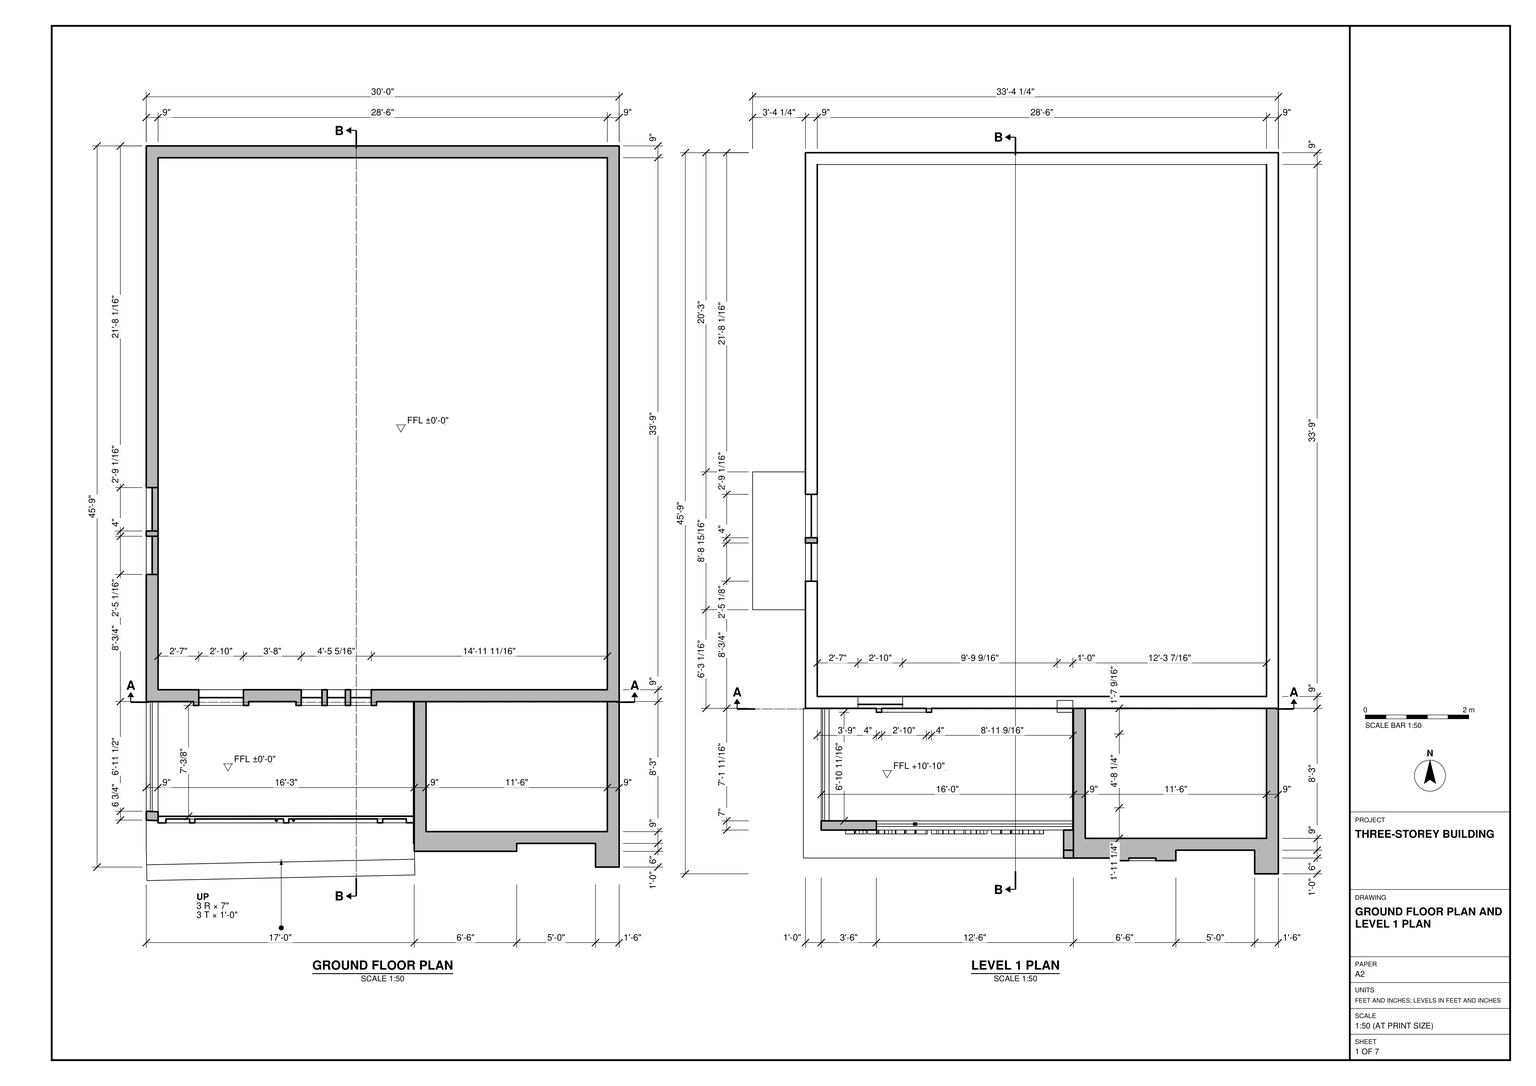
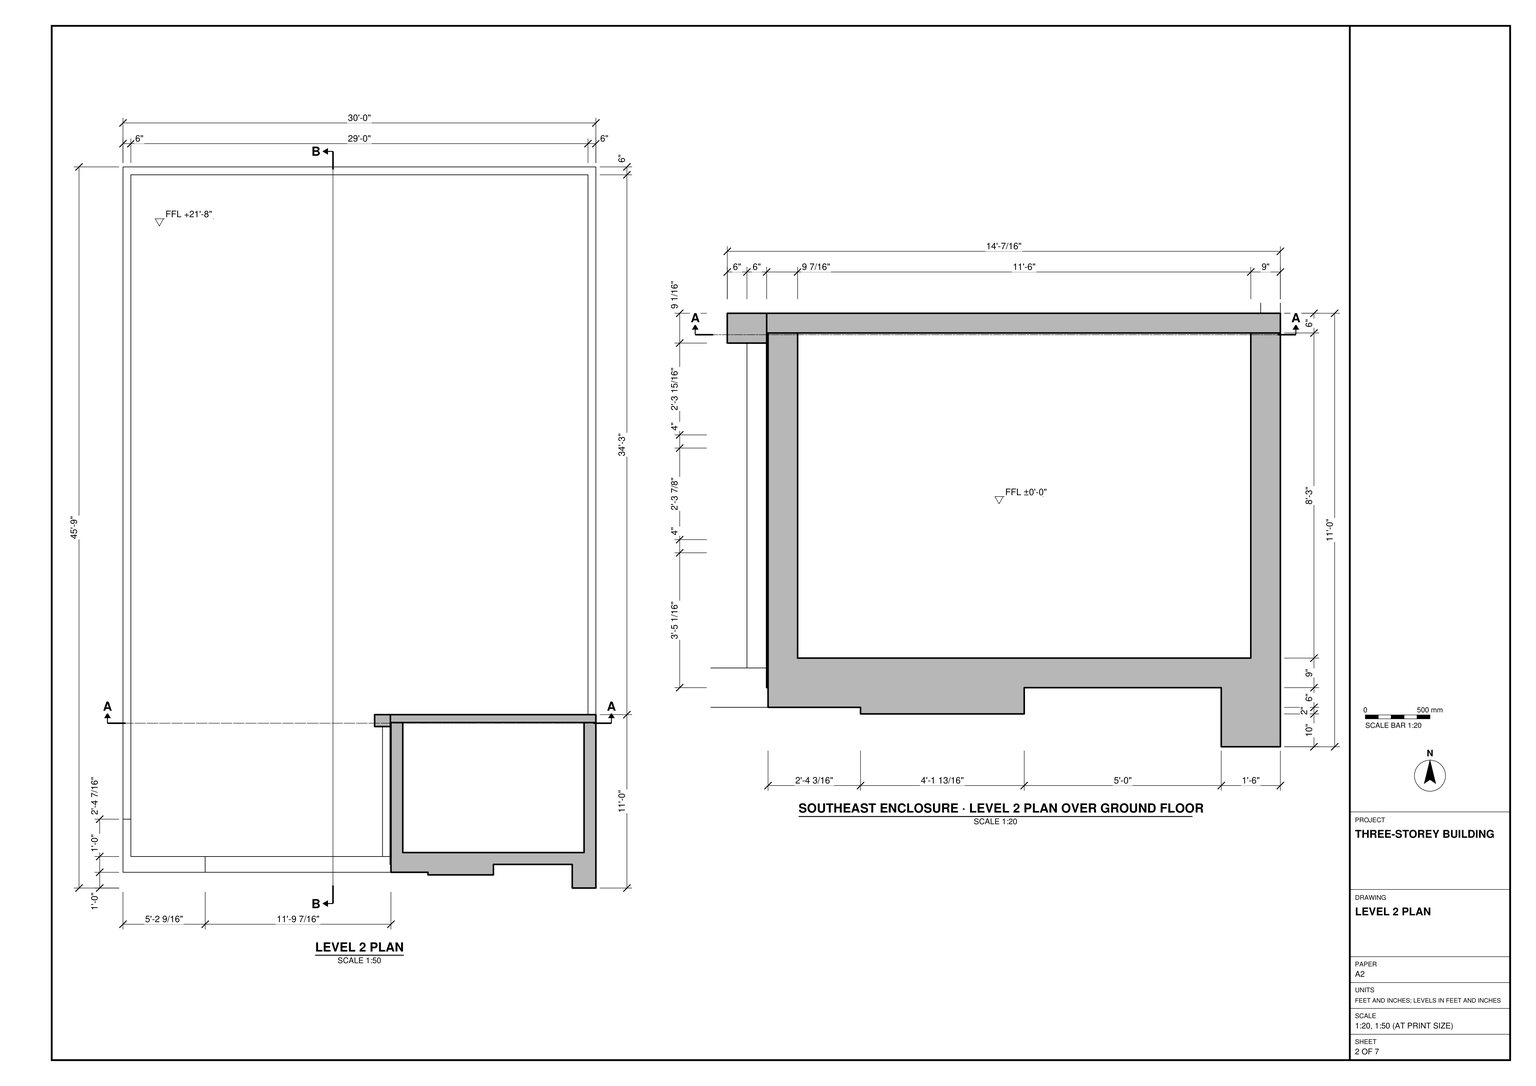
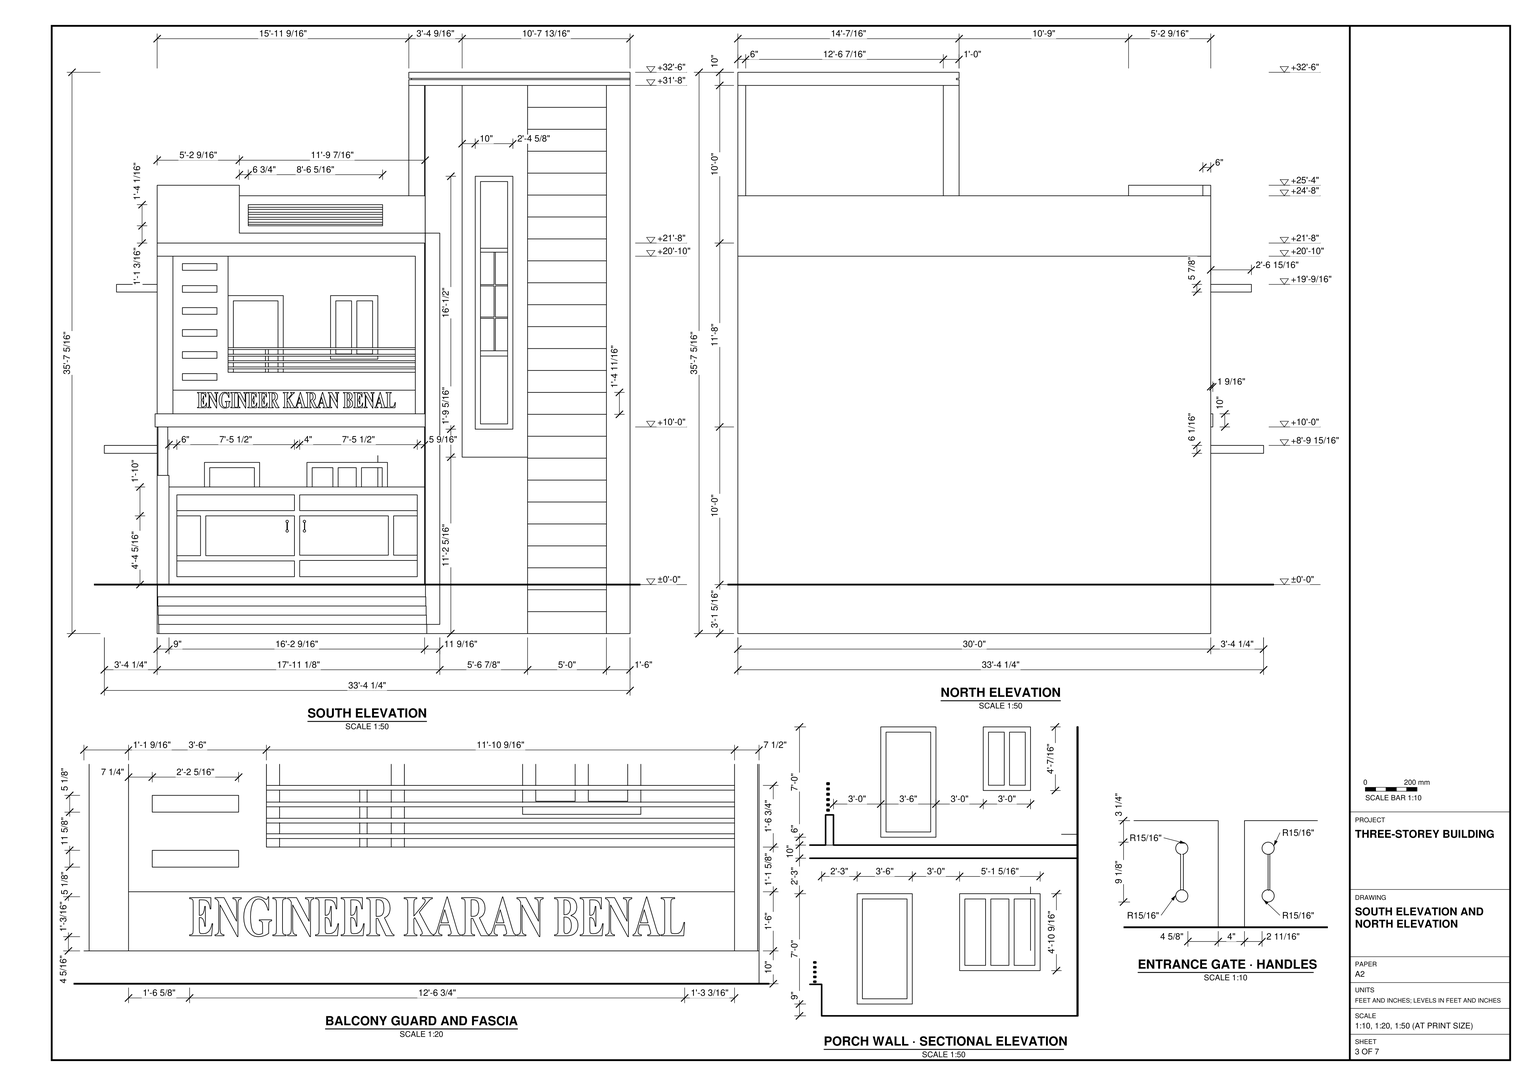
Build the three-storey building in SketchUp from task_files/diagram_01.pdf. Work in feet and inches. The complete model measures 33'-4 1/4" east to west, 49'-7 1/4" north to south and 35'-7 5/16" from the bottom of the base to the top of the roof. Set the ground floor at ±0'-0", Level 1 at +10'-0" and Level 2 at +21'-8".

Use the plans to lay out the rectangular main floor plates and the two bays on the south front. Keep the main floor areas open as drawn. Model the base, floor slabs, exterior walls, side projections and framed openings, using the wall thicknesses shown. In the western bay, build the entrance steps, double-leaf gate and covered porch. Place the balcony above the porch, with its solid fascia, horizontal guard rails and slotted end screen. Set the doors and windows in the walls behind the porch and balcony. In the eastern bay, carry the enclosure up past the terrace and reproduce the tall framed opening and adjacent horizontal joints on its south face. Finish the terrace with its parapets and the taller enclosure with its projecting flat roof cap.

Keep walls, slabs, roofs and each furniture or joinery piece shown in separate groups or components, and use components for repeated parts. Any decor or loose items shown may be suitable library components. Save one SketchUp model as output_files/three_storey_building_with_a_porch_and_roof_terrace.skp.

# SketchUp Ruby script. Lengths in inches.
U = 1.inch
M = Sketchup.active_model
def pt(a) = Geom::Point3d.new(a.map { |v| v * U })
def face(e, loops, mat)
  f = e.add_face(loops[0].map { |a| pt(a) })
  loops[1..].each { |l| e.add_face(l.map { |a| pt(a) }).erase! }
  f.material = f.back_material = mat if mat
  f
end
# faces: each face lists its corners as indices into pts; further lists are holes
def faces(e, pts, list, mat = nil) = list.each { |f| face(e, (f[0].is_a?(Array) ? f : [f]).map { |l| l.map { |i| pts[i] } }, mat) }
# xy, xz, yz: faces in a plane at the given z, y or x. An outline is a flat list of corners, or four numbers for a rectangle; further outlines are holes
def ring(l) = l.size == 4 ? [[l[0], l[1]], [l[2], l[1]], [l[2], l[3]], [l[0], l[3]]] : l.each_slice(2).to_a
def flat(e, list, mat, &to3) = list.each { |f| face(e, (f[0].is_a?(Array) ? f : [f]).map { |l| ring(l).map { |u, v| to3.(u, v) } }, mat) }
def xy(e, z, list, mat = nil) = flat(e, list, mat) { |x, y| [x, y, z] }
def xz(e, y, list, mat = nil) = flat(e, list, mat) { |x, z| [x, y, z] }
def yz(e, x, list, mat = nil) = flat(e, list, mat) { |y, z| [x, y, z] }
def lines(e, pts, list) = list.each { |a, b| e.add_line(pt(pts[a]), pt(pts[b])) }
# prism: a flat outline (further loops are holes) pulled along v
def prism(e, loops, v, mat = nil)
  f = face(e, loops, mat); d = Geom::Vector3d.new(v.map { |x| x * U })
  f.pushpull(f.normal.samedirection?(d) ? d.length : -d.length)
end
def box(e, o, s, mat = nil) = prism(e, [[o, [o[0] + s[0], o[1], o[2]], [o[0] + s[0], o[1] + s[1], o[2]], [o[0], o[1] + s[1], o[2]]]], [0, 0, s[2]], mat)
def at(x, y, z, deg = 0) = Geom::Transformation.translation(pt([x, y, z])) * Geom::Transformation.rotation(ORIGIN, Z_AXIS, deg.degrees)
def axes(o, x, y, z) = Geom::Transformation.new([*x, 0, *y, 0, *z, 0, *pt(o).to_a, 1])
def part(name) = M.definitions.add(name)
# library, detail: a bought-in or finely detailed component or shape, given as its bounding box
def library(name, o, s) = part(name).tap { |d| box(d.entities, o, s) }
def detail(e, o, s) = box(e.add_group.entities, o, s)
def put(e, d, t, mat = nil) = e.add_instance(d, t).tap { |i| i.material = mat if mat }
def group(e, t, mat = nil) = e.add_group.tap { |g| g.transformation = t; g.material = mat if mat }.entities
root = M.entities
M.materials.add("B01_Ivory_Dust").color = [255, 217, 206]
M.materials.add("B02_Almond_Blush").color = [255, 177, 153]
M.materials.add("D07_Ochre_Flame").color = [146, 133, 153]
M.materials.add("Glass_Mirror_01").color = [185, 155, 104]
M.materials.add("Glass_Mirror_1").color = [185, 154, 113]
M.materials.add("Glass_Mirror_2").color = [185, 185, 185]
M.materials.add("Metal_Perforated_08_1K").color = [255, 203, 117]
M.materials.add("Wood_Floor_12_1K").color = [92, 75, 65]
M.materials.add("Wood_Planks_01_1K").color = [69, 67, 63]
M.materials.add("Wood_Veneer_15_1K").color = [142, 95, 62]
M.materials.add("Wood_Veneer_15_1K1").color = [103, 69, 45]
c1 = library("ENGINEER KARAN B",[0.35,0,0],[228.41,12.29,1])
xy(root,-27.305,[[41.498,0,40.236,59.987,244.236,64.279,244.236,58.279,244.363,58.279,245.498,4.292],[382.236,46.279,382.236,64.279,322.236,64.279,322.236,58.279,244.363,58.279,244.236,64.279,40.236,59.987,40.236,595.279,400.236,595.279,400.236,46.279],[244.236,58.279,244.236,64.279,244.363,58.279]])
xy(root,-20.305,[[41.498,0,245.498,4.292,245.246,16.289,41.246,11.997],[244.236,58.279,244.363,58.279,244.236,64.279]])
xy(root,-13.305,[[41.246,11.997,245.246,16.289,244.994,28.287,40.994,23.995]])
xy(root,-6.305,[[40.994,23.995,244.994,28.287,244.741,40.284,40.741,35.992]])
xy(root,0.695,[[40.741,35.992,244.741,40.284,244.489,52.282,40.489,47.989]])
xy(root,10,[[40.489,47.989,244.489,52.282,244.363,58.279,244.236,64.279,243.811,64.279,243.812,79.984,243.812,82.984,243.811,84.984,49.236,84.893,49.236,81.612,40.236,82.023,40.236,59.987],[243.811,64.279,243.812,79.984,244.237,79.984,244.236,64.279],[253.236,73.279,391.236,172.279],[49.239,79.893,49.236,84.893,243.811,84.984,243.812,82.984,243.812,79.984],[243.812,79.984,244.237,82.984],
  [244.237,79.984,244.237,82.984,244.239,79.984],[243.812,82.984,243.811,84.984,244.236,84.984,244.237,82.984],[49.236,84.893,243.811,84.984,49.236,84.984],[49.236,84.984,243.811,172.279],[243.811,84.984,244.236,172.279],
  [49.236,181.279,391.236,586.279]])
xy(root,16,[[55.239,79.896,144.739,79.938,144.737,82.938,55.237,82.896],[148.739,79.94,238.239,79.981,238.237,82.981,148.737,82.94]])
xy(root,19,[[76.236,169.279,118.236,172.279]])
xy(root,23,[[80.236,175.279,114.236,181.279]])
xy(root,23,[[80.236,169.279,114.236,175.279]],"Wood_Floor_12_1K")
xy(root,28,[[55.239,79.896,55.237,82.896,144.737,82.938,144.739,79.938]])
xy(root,28.369,[[148.739,79.94,148.737,82.94,238.237,82.981,238.239,79.981]])
xy(root,32,[[55.239,79.896,73.239,79.904,73.237,82.904,55.237,82.896],[77.239,79.906,144.739,79.938,144.737,82.938,77.237,82.906]])
xy(root,32.369,[[148.739,79.94,216.239,79.971,216.237,82.971,148.737,82.94],[220.239,79.973,238.239,79.981,238.237,82.981,220.237,82.973]])
xy(root,34,[[49.236,88.357,49.236,172.279,40.236,172.279,40.236,88.768]])
xy(root,35.574,[[43.299,88.661,44.778,172.279]],"Wood_Planks_01_1K")
xy(root,35.696,[[44.736,269.04,49.236,298.119],[44.736,302.119,49.236,335.198]])
xy(root,35.696,[[40.236,269.04,44.736,298.119],[40.236,302.119,44.736,335.198]],"Wood_Planks_01_1K")
xy(root,36.363,[[43.299,88.661,44.778,172.279]],"Wood_Planks_01_1K")
xy(root,39.256,[[43.299,88.661,44.778,172.279]],"Wood_Planks_01_1K")
xy(root,40.045,[[43.299,88.661,44.778,172.279]],"Wood_Planks_01_1K")
xy(root,42.938,[[43.299,88.661,44.778,172.279]],"Wood_Planks_01_1K")
xy(root,43.727,[[43.299,88.661,44.778,172.279]],"Wood_Planks_01_1K")
xy(root,44.433,[[154.236,169.279,215.556,172.279]])
xy(root,46.62,[[43.299,88.661,44.778,172.279]],"Wood_Planks_01_1K")
xy(root,47.409,[[43.299,88.661,44.778,172.279]])
xy(root,48.433,[[158.236,175.279,174.01,181.279],[178.01,175.279,191.783,181.279],[195.783,175.279,211.556,181.279]])
xy(root,48.433,[[158.236,169.279,174.01,175.279],[178.01,169.279,191.783,175.279],[195.783,169.279,211.556,175.279]],"Wood_Veneer_15_1K1")
xy(root,50.302,[[43.299,88.661,44.778,172.279]],"Wood_Planks_01_1K")
xy(root,51.09,[[43.299,88.661,44.778,172.279]])
xy(root,62.301,[[55.239,79.896,55.237,82.896,73.237,82.904,73.239,79.904],[77.239,79.906,77.237,82.906,144.737,82.938,144.739,79.938],[148.739,79.94,148.737,82.94,216.237,82.971,216.239,79.971],[220.239,79.973,220.237,82.973,238.237,82.981,238.239,79.981]])
xy(root,66.301,[[55.239,79.896,144.739,79.938,144.737,82.938,55.237,82.896],[148.739,79.94,238.239,79.981,238.237,82.981,148.737,82.94]])
xy(root,78.301,[[55.239,79.896,55.237,82.896,144.737,82.938,144.739,79.938],[144.739,79.938,144.737,82.938,148.737,82.94,148.739,79.94],[148.739,79.94,148.737,82.94,238.237,82.981,238.239,79.981]])
xy(root,84.301,[[49.239,79.893,244.239,79.984,244.236,84.984,49.236,84.893]])
xy(root,93.11,[[[49.236,81.612,49.236,88.357,40.236,88.768,40.236,82.023,40.884,81.993],[40.884,81.993,48.316,87.588]]])
xy(root,99,[[80.236,175.279,114.236,181.279],[158.236,175.279,174.01,181.279],[178.01,175.279,191.783,181.279],[195.783,175.279,211.556,181.279]])
xy(root,99,[[80.236,169.279,114.236,175.279]],"Wood_Floor_12_1K")
xy(root,99,[[158.236,169.279,174.01,175.279],[178.01,169.279,191.783,175.279],[195.783,169.279,211.556,175.279]],"Wood_Veneer_15_1K1")
xy(root,103,[[76.236,169.279,118.236,172.279],[154.236,169.279,215.556,172.279]])
xy(root,104.327,[[40.236,269.04,44.736,298.119],[44.736,269.04,49.236,298.119],[40.236,302.119,44.736,335.198],[44.736,302.119,49.236,335.198]])
xy(root,106.994,[[272.399,56.279,322.236,58.279]])
xy(root,109.906,[[0,247.314,40.236,352.29]])
xy(root,115.954,[[0,247.314,40.236,352.29]])
xy(root,130,[[[38.65,58.279,244.236,172.279],[40.884,81.993,48.316,87.588]],[40.884,81.993,48.316,87.588]])
xy(root,132.316,[[286.379,56.279,307.017,58.279]])
xy(root,140,[[38.65,58.279,236.767,58.279,236.767,79.59,52.236,79.59,52.236,172.279,38.65,172.279],[236.767,58.279,244.236,64.279],[236.767,64.279,243.811,79.59],[236.767,64.279,244.236,79.59],[243.811,64.279,244.236,79.59],
  [58.236,86.59,244.236,172.279]])
xy(root,146,[[94.236,169.279,136.236,172.279]])
xy(root,148.205,[[231.811,169.208,243.811,178.279]])
xy(root,150,[[98.236,169.279,132.236,172.279]],"Wood_Floor_12_1K")
xy(root,157.491,[[44.736,269.04,49.236,298.119],[44.736,302.119,49.236,335.198]])
xy(root,157.491,[[40.236,269.04,44.736,298.119],[40.236,302.119,44.736,335.198]],"Wood_Planks_01_1K")
xy(root,163.013,[[52.236,86.59,58.236,172.279]])
xy(root,165.505,[[59.46,79.59,85.759,86.59]])
xy(root,166.058,[[53.305,86.544,54.875,172.279]])
xy(root,167.202,[[53.305,86.544,54.875,172.279]])
xy(root,170.084,[[53.305,86.544,54.875,172.279]])
xy(root,170.613,[[59.46,79.59,85.759,86.59]])
xy(root,171.227,[[53.305,86.544,54.875,172.279]])
xy(root,171.618,[[[94.223,79.59,244.236,86.59],[122.643,83.502,124.887,84.898]],[122.643,83.502,124.887,84.898]])
xy(root,174.109,[[53.305,86.544,54.875,172.279]])
xy(root,174.219,[[94.223,82.305,244.591,84.229]])
xy(root,175.253,[[53.305,86.544,54.875,172.279]])
xy(root,175.658,[[94.223,82.305,244.591,84.229]])
xy(root,178.134,[[53.305,86.544,54.875,172.279]])
xy(root,178.941,[[94.223,82.305,244.591,84.229]])
xy(root,179.278,[[53.305,86.544,54.875,172.279]])
xy(root,180.381,[[94.223,82.305,244.591,84.229]])
xy(root,181.575,[[172.236,169.279,208.236,172.279]])
xy(root,182.16,[[53.305,86.544,54.875,172.279]])
xy(root,182.253,[[59.46,79.59,85.759,86.59]])
xy(root,183.303,[[53.305,86.544,54.875,172.279]])
xy(root,183.875,[[94.223,82.305,244.591,84.229]])
xy(root,183.975,[[286.379,56.279,307.017,58.279]])
xy(root,185.315,[[94.223,82.305,244.591,84.229]])
xy(root,185.575,[[176.236,169.279,188.236,172.279],[192.236,169.279,204.236,172.279]],"Wood_Veneer_15_1K1")
xy(root,186.185,[[53.305,86.544,54.875,172.279]])
xy(root,187.329,[[53.305,86.544,54.875,172.279]])
xy(root,187.361,[[59.46,79.59,85.759,86.59]])
xy(root,187.975,[[286.379,56.279,296.698,58.279],[297.698,56.279,307.017,58.279]])
xy(root,188.951,[[94.223,82.305,244.591,84.229]])
xy(root,190.031,[[122.643,83.502,124.887,84.898]])
xy(root,190.391,[[94.223,82.305,244.591,84.229]])
xy(root,199.001,[[59.46,79.59,85.759,86.59]])
xy(root,204.109,[[59.46,79.59,85.759,86.59]])
xy(root,212.665,[[286.379,56.279,296.698,58.279],[297.698,56.279,307.017,58.279]])
xy(root,213.665,[[286.379,56.279,296.698,58.279],[297.698,56.279,307.017,58.279],[297.698,58.279,307.017,60.797]])
xy(root,215.749,[[59.46,79.59,85.759,86.59]])
xy(root,220.857,[[59.46,79.59,85.759,86.59]])
xy(root,226,[[98.236,169.279,132.236,172.279],[176.236,169.279,188.236,172.279],[192.236,169.279,204.236,172.279]])
xy(root,226.123,[[40.236,269.04,44.736,298.119],[44.736,269.04,49.236,298.119],[40.236,302.119,44.736,335.198],[44.736,302.119,49.236,335.198]])
xy(root,230,[[94.236,169.279,136.236,172.279]])
xy(root,230,[[172.236,169.279,208.236,172.279]],"Wood_Veneer_15_1K1")
xy(root,232.497,[[59.46,79.59,85.759,86.59]])
xy(root,232.695,[[9.275,242.247,40.236,352.542]])
xy(root,237.355,[[286.379,56.279,296.698,58.279],[297.698,56.279,307.017,58.279],[297.698,58.279,307.017,60.797]])
xy(root,237.605,[[59.46,79.59,85.759,86.59]])
xy(root,238.355,[[286.379,56.279,296.698,58.279],[297.698,56.279,307.017,56.622],[297.698,56.622,307.017,58.279],[297.698,58.279,307.017,59.028]])
xy(root,238.545,[[21.275,242.247,40.236,242.247,40.236,352.542,9.275,352.542,9.275,263.238,9.281,262.861,9.299,262.484,9.329,262.108,9.37,261.734,9.423,261.361,9.488,260.989,9.564,260.62,9.652,260.254,9.752,259.89,9.863,259.53,9.985,259.173,10.118,258.82,10.262,258.472,10.417,258.128,10.583,257.79,10.76,257.457,10.946,257.129,11.143,256.808,11.35,256.493,11.567,256.184,11.793,255.883,12.029,255.589,12.274,255.302,12.528,255.023,12.79,254.753,13.061,254.49,13.34,254.236,13.626,253.992,13.92,253.756,14.222,253.53,14.53,253.313,14.845,253.106,15.167,252.909,15.494,252.722,15.827,252.546,16.166,252.38,16.51,252.225,16.858,252.08,17.21,251.947,17.567,251.825,17.927,251.714,18.291,251.615,18.658,251.527,19.027,251.45,19.398,251.386,19.771,251.332,20.146,251.291,20.522,251.261,20.898,251.244,21.275,251.238],[9.275,242.247,21.275,242.247,21.275,251.238,20.898,251.244,20.522,251.261,20.146,251.291,19.771,251.332,19.398,251.386,19.027,251.45,18.658,251.527,18.291,251.615,17.927,251.714,17.567,251.825,17.21,251.947,16.858,252.08,16.51,252.225,16.166,252.38,15.827,252.546,15.494,252.722,15.167,252.909,14.845,253.106,14.53,253.313,14.222,253.53,13.92,253.756,13.626,253.992,13.34,254.236,13.061,254.49,12.79,254.753,12.528,255.023,12.274,255.302,12.029,255.589,11.793,255.883,11.567,256.184,11.35,256.493,11.143,256.808,10.946,257.129,10.76,257.457,10.583,257.79,10.417,258.128,10.262,258.472,10.118,258.82,9.985,259.173,9.863,259.53,9.752,259.89,9.652,260.254,9.564,260.62,9.488,260.989,9.423,261.361,9.37,261.734,9.329,262.108,9.299,262.484,9.281,262.861,9.275,263.238]])
xy(root,249.245,[[59.46,79.59,85.759,86.59]])
xy(root,254.353,[[59.46,79.59,85.759,86.59]])
xy(root,260,[[40.236,58.279,236.767,64.279],[236.767,64.279,244.236,79.59],[243.811,64.279,244.236,79.59],[52.236,79.59,94.223,86.59],[[40.236,172.279,400.236,595.279],[49.236,181.279,391.236,586.279]]])
xy(root,263.045,[[286.379,56.279,296.698,58.279],[297.698,56.279,307.017,56.622],[297.698,56.622,307.017,58.279],[297.698,58.279,307.017,59.028]])
xy(root,266.045,[[286.379,56.279,307.017,58.279]])
xy(root,270,[[40.236,58.279,244.236,64.279],[231.811,169.208,243.811,178.279]])
xy(root,316.84,[[286.379,56.279,307.017,58.279]])
xy(root,390,[[231.811,46.279,231.811,169.208,243.811,169.208,243.811,64.279,244.236,64.279,244.236,58.279,272.399,58.279,272.399,56.279,322.236,56.279,322.236,64.279,382.236,64.279,382.236,46.279],[382.236,46.279,400.236,64.279],[272.399,56.279,322.236,64.279],[244.236,58.279,272.399,64.279],[243.811,64.279,243.811,178.279,400.236,178.279,400.236,172.279,244.236,172.279,244.236,64.279],
  [243.811,64.279,244.236,172.279],[244.236,64.279,244.236,172.279,253.236,172.279,253.236,73.279,391.236,73.279,391.236,172.279,400.236,172.279,400.236,64.279],[253.236,73.279,391.236,172.279],[253.236,73.279,391.236,172.279],[231.811,169.208,243.811,178.279]])
xy(root,394.4,[[231.811,46.279,400.236,47.303],[231.811,47.303,233.885,178.279]])
xy(root,395.4,[[231.811,46.279,400.236,47.303],[231.811,47.303,233.885,178.279]])
xy(root,400,[[231.811,46.279,400.236,178.279]])
xz(root,46.279,[[382.236,-27.305,400.236,390],[231.811,390,400.236,394.4],[231.811,395.4,400.236,400]])
xz(root,47.303,[[233.885,394.4,400.236,395.4]])
xz(root,56.279,[[[282.379,128.316,311.017,320.84],[286.379,132.316,307.017,316.84]],[286.379,183.975,307.017,187.975],[296.698,187.975,297.698,187.975,297.698,212.665,307.017,212.665,307.017,213.665,297.698,213.665,297.698,237.355,307.017,237.355,307.017,238.355,297.698,238.355,297.698,263.045,296.698,263.045,296.698,238.355,286.379,238.355,286.379,237.355,296.698,237.355,296.698,213.665,286.379,213.665,286.379,212.665,296.698,212.665],[286.379,263.045,307.017,266.045]])
xz(root,56.279,[[[272.399,106.994,322.236,390],[282.379,128.316,311.017,320.84]]],"D07_Ochre_Flame")
xz(root,58.279,[[244.236,-27.305,322.236,-27.305,322.236,106.994,272.399,106.994,272.399,390,244.236,390,244.236,277.559,255.386,277.559,255.386,-20.305,244.236,-20.305],[38.65,130,244.236,140],[236.767,140,243.811,140,243.811,270,40.236,270,40.236,260,236.767,260],[243.811,140,244.236,270]])
xz(root,58.279,[[286.379,132.316,307.017,183.975],[286.379,266.045,307.017,316.84]],"B02_Almond_Blush")
xz(root,58.279,[[244.236,-20.305,255.386,-20.305,255.386,277.559,244.236,277.559,244.363,270,244.363,-17.476,244.236,277.559],[244.363,-17.476,244.363,270,244.236,277.559]],"D07_Ochre_Flame")
xz(root,58.279,[[286.379,187.975,296.698,212.665],[297.698,187.975,307.017,212.665],[286.379,213.665,296.698,237.355],[297.698,213.665,307.017,237.355],[286.379,238.355,296.698,263.045],
  [297.698,238.355,307.017,263.045]],"Glass_Mirror_1")
xz(root,60.797,[[297.698,213.665,307.017,237.355]])
xz(root,64.279,[[243.811,10,244.236,140],[236.767,140,243.811,260],[243.811,140,244.236,260],[40.236,260,243.811,270],[243.811,260,244.236,270],
  [243.811,270,244.236,390]])
xz(root,64.279,[[322.236,-27.305,382.236,-10.613],[322.236,-10.613,382.236,6.08],[322.236,6.08,382.236,22.772],[322.236,22.772,382.236,39.464],[322.236,39.464,382.236,56.156],
  [322.236,56.156,382.236,72.848],[322.236,72.848,382.236,89.54],[322.236,89.54,382.236,106.233],[322.236,106.233,382.236,122.925],[322.236,122.925,382.236,139.617],
  [322.236,139.617,382.236,156.309],[322.236,156.309,382.236,173.001],[322.236,173.001,382.236,189.694],[322.236,189.694,382.236,206.386],[322.236,206.386,382.236,223.078],
  [322.236,223.078,382.236,239.77],[322.236,239.77,382.236,256.462],[322.236,256.462,382.236,273.155],[322.236,273.155,382.236,289.847],[322.236,289.847,382.236,306.539],
  [322.236,306.539,382.236,323.231],[322.236,323.231,382.236,339.923],[322.236,339.923,382.236,356.616],[322.236,356.616,382.236,373.308],[322.236,373.308,382.236,390]],"D07_Ochre_Flame")
xz(root,73.279,[[253.236,10,391.236,390]])
xz(root,79.59,[[236.767,140,243.811,158],[[52.236,158,236.767,158,236.767,171.618,94.223,171.618,94.223,260,52.236,260],[59.46,165.505,85.759,170.613],[59.46,249.245,85.759,254.353],[59.46,182.253,85.759,187.361],[59.46,199.001,85.759,204.109],[59.46,215.749,85.759,220.857],[59.46,232.497,85.759,237.605]],[236.767,158,243.811,171.618],[243.811,158,244.236,171.618],[236.767,171.618,243.811,260]])
xz(root,79.59,[[52.236,140,236.767,158],[236.767,140,244.236,158]],"D07_Ochre_Flame")
xz(root,80.752,[[139.431,51.726,139.431,57.204,139.31,57.173,139.067,57.174,139.007,57.19,139.007,51.74,139.077,51.758,139.32,51.757]])
xz(root,81.347,[[139.431,51.726,139.32,51.757,139.076,51.758,139.007,51.74,139.007,57.19,139.067,57.174,139.31,57.173,139.431,57.204]])
xz(root,81.993,[[40.884,93.11,48.316,130]])
xz(root,82.305,[[94.223,174.219,244.591,175.658],[94.223,178.941,244.591,180.381],[94.223,183.875,244.591,185.315],[94.223,188.951,244.591,190.391]])
xz(root,83.502,[[122.643,171.618,124.887,190.031]])
xz(root,84.229,[[94.223,174.219,244.591,175.658],[94.223,178.941,244.591,180.381],[94.223,183.875,244.591,185.315],[94.223,188.951,244.591,190.391]])
xz(root,84.898,[[122.643,171.618,124.887,190.031]])
xz(root,86.544,[[53.305,166.058,54.875,167.202],[53.305,170.084,54.875,171.227],[53.305,174.109,54.875,175.253],[53.305,178.134,54.875,179.278],[53.305,182.16,54.875,183.303],
  [53.305,186.185,54.875,187.329]])
xz(root,86.59,[[[58.236,140,58.236,260,94.223,260,94.223,171.618,244.236,171.618,244.236,140],[59.46,165.505,85.759,170.613],[59.46,182.253,85.759,187.361],[59.46,199.001,85.759,204.109],[59.46,215.749,85.759,220.857],[59.46,232.497,85.759,237.605],[59.46,249.245,85.759,254.353]],[52.236,163.013,58.236,260]])
xz(root,87.588,[[40.884,93.11,48.316,130]])
xz(root,88.661,[[43.299,35.574,44.778,36.363]])
xz(root,169.208,[[231.811,270,243.811,390]])
xz(root,169.279,[[[76.236,19,118.236,103],[80.236,23,114.236,99]],[[94.236,146,136.236,230],[98.236,150,132.236,226]]],"Wood_Floor_12_1K")
xz(root,169.279,[[[154.236,44.433,215.556,103],[195.783,48.433,211.556,99],[158.236,48.433,174.01,99],[178.01,48.433,191.783,99]],[[172.236,181.575,208.236,230],[176.236,185.575,188.236,226],[192.236,185.575,204.236,226]]],"Wood_Veneer_15_1K1")
xz(root,172.279,[[391.236,8.205,400.236,10],[[49.236,10,243.811,10,243.811,130,40.236,130,40.236,34,49.236,34],[154.236,44.433,215.556,103],[76.236,19,118.236,103],[43.299,35.574,44.778,36.363]],[243.811,10,244.236,18.205],[244.236,10,253.236,18.205],[253.236,10,391.236,18.205],
  [391.236,10,400.236,18.205],[243.811,18.205,244.236,130],[243.811,18.205,244.236,138.205],[244.236,18.205,253.236,130],[253.236,18.205,391.236,130],
  [391.236,18.205,400.236,130],[38.65,130,40.236,140],[243.811,130,253.236,390],[244.236,130,253.236,138.205],[253.236,130,391.236,138.205],
  [391.236,130,400.236,138.205],[244.236,138.205,253.236,140],[253.236,138.205,391.236,140],[391.236,138.205,400.236,140],[[40.236,140,40.236,260,243.811,260,243.811,140,58.236,140,58.236,163.013,52.236,163.013,52.236,140],[94.236,146,136.236,230],[172.236,181.575,208.236,230],[53.305,166.058,54.875,167.202],[53.305,170.084,54.875,171.227],[53.305,174.109,54.875,175.253],[53.305,178.134,54.875,179.278],[53.305,182.16,54.875,183.303],[53.305,186.185,54.875,187.329]],
  [52.236,140,58.236,163.013],[243.811,140,244.236,260],[244.236,140,253.236,260],[253.236,140,391.236,260],[391.236,140,400.236,260],
  [53.305,166.058,54.875,167.202],[53.305,170.084,54.875,171.227],[53.305,174.109,54.875,175.253],[53.305,178.134,54.875,179.278],[53.305,182.16,54.875,183.303],
  [53.305,186.185,54.875,187.329],[391.236,260,400.236,390]])
xz(root,172.279,[[98.236,150,132.236,226],[176.236,185.575,188.236,226],[192.236,185.575,204.236,226]],"Glass_Mirror_1")
xz(root,175.279,[[80.236,153,114.236,229],[158.236,179.127,173.236,229],[177.236,179.127,192.236,229]])
xz(root,175.279,[[80.236,23,114.236,99],[158.236,48.433,174.01,99],[178.01,48.433,191.783,99],[195.783,48.433,211.556,99]],"Glass_Mirror_1")
xz(root,178.279,[[231.811,270,243.811,390],[231.811,390,231.811,394.4,233.885,394.4,233.885,395.4,231.811,395.4,231.811,400,400.236,400,400.236,390]])
xz(root,181.279,[[[49.236,10,391.236,130],[80.236,23,114.236,99],[195.783,48.433,211.556,99],[158.236,48.433,174.01,99],[178.01,48.433,191.783,99]],[[49.236,140,391.236,260],[158.236,179.127,173.236,229]]])
xz(root,242.247,[[9.275,232.695,40.236,238.545]])
xz(root,247.314,[[0,109.906,40.236,115.954]])
xz(root,269.04,[[44.736,35.696,49.236,104.327],[44.736,157.491,49.236,226.123]])
xz(root,269.04,[[40.236,35.696,44.736,104.327],[40.236,157.491,44.736,226.123]],"Wood_Planks_01_1K")
xz(root,298.119,[[44.736,35.696,49.236,104.327],[44.736,157.491,49.236,226.123]])
xz(root,298.119,[[40.236,35.696,44.736,104.327],[40.236,157.491,44.736,226.123]],"Wood_Planks_01_1K")
xz(root,302.119,[[44.736,35.696,49.236,104.327],[44.736,157.491,49.236,226.123]])
xz(root,302.119,[[40.236,35.696,44.736,104.327],[40.236,157.491,44.736,226.123]],"Wood_Planks_01_1K")
xz(root,335.198,[[44.736,35.696,49.236,104.327],[44.736,157.491,49.236,226.123]])
xz(root,335.198,[[40.236,35.696,44.736,104.327],[40.236,157.491,44.736,226.123]],"Wood_Planks_01_1K")
xz(root,352.29,[[0,109.906,40.236,115.954]])
xz(root,352.542,[[9.275,232.695,40.236,238.545]])
xz(root,586.279,[[49.236,10,391.236,130]])
xz(root,595.279,[[40.236,-27.305,400.236,260]])
yz(root,0,[[247.314,109.906,352.29,115.954]])
yz(root,9.275,[[242.247,232.695,352.542,238.545]])
yz(root,38.65,[[58.279,130,172.279,140]])
yz(root,40.236,[[[59.987,-27.305,59.987,10,88.768,10,88.768,34,172.279,34,172.279,260,595.279,260,595.279,-27.305],[265.04,153.491,339.198,230.123],[265.04,31.696,339.198,108.327],[242.247,232.695,352.542,238.545],[247.314,109.906,352.29,115.954]],[58.279,260,64.279,270]])
yz(root,40.236,[[82.023,10,88.768,93.11]],"D07_Ochre_Flame")
yz(root,40.236,[[[265.04,31.696,339.198,108.327],[269.04,35.696,335.198,104.327]],[298.119,35.696,302.119,104.327],[[265.04,153.491,339.198,230.123],[269.04,157.491,335.198,226.123]],[298.119,157.491,302.119,226.123]],"Wood_Planks_01_1K")
yz(root,40.884,[[81.993,93.11,87.588,130]])
yz(root,43.299,[[88.661,35.574,172.279,36.363],[88.661,39.256,172.279,40.045],[88.661,42.938,172.279,43.727],[88.661,46.62,172.279,47.409],[88.661,50.302,172.279,51.09]],"Wood_Planks_01_1K")
yz(root,44.736,[[269.04,35.696,298.119,104.327],[302.119,35.696,335.198,104.327],[269.04,157.491,298.119,226.123],[302.119,157.491,335.198,226.123]],"Glass_Mirror_2")
yz(root,44.778,[[88.661,39.256,172.279,40.045],[88.661,42.938,172.279,43.727],[88.661,46.62,172.279,47.409],[88.661,50.302,172.279,51.09]])
yz(root,44.778,[[88.661,35.574,172.279,36.363]],"Wood_Planks_01_1K")
yz(root,48.316,[[81.993,93.11,87.588,130]])
yz(root,49.236,[[88.357,10,172.279,34],[181.279,10,586.279,130],[[181.279,140,586.279,260],[302.119,157.491,335.198,226.123],[269.04,157.491,298.119,226.123]]])
yz(root,49.236,[[81.612,10,88.357,93.11]],"D07_Ochre_Flame")
yz(root,52.236,[[79.59,140,79.59,260,86.59,260,86.59,163.013,172.279,163.013,172.279,140]])
yz(root,53.305,[[86.544,166.058,172.279,167.202],[86.544,170.084,172.279,171.227],[86.544,174.109,172.279,175.253],[86.544,178.134,172.279,179.278],[86.544,182.16,172.279,183.303],
  [86.544,186.185,172.279,187.329]])
yz(root,54.875,[[86.544,166.058,172.279,167.202],[86.544,170.084,172.279,171.227],[86.544,174.109,172.279,175.253],[86.544,178.134,172.279,179.278],[86.544,182.16,172.279,183.303],
  [86.544,186.185,172.279,187.329]])
yz(root,58.236,[[86.59,140,172.279,163.013]])
yz(root,59.46,[[79.59,165.505,86.59,170.613],[79.59,182.253,86.59,187.361],[79.59,199.001,86.59,204.109],[79.59,215.749,86.59,220.857],[79.59,232.497,86.59,237.605],
  [79.59,249.245,86.59,254.353]])
yz(root,76.236,[[169.279,19,172.279,103]],"Wood_Floor_12_1K")
yz(root,80.236,[[175.279,23,181.279,99]])
yz(root,80.236,[[169.279,23,175.279,99]],"Wood_Floor_12_1K")
yz(root,85.759,[[79.59,165.505,86.59,170.613],[79.59,182.253,86.59,187.361],[79.59,199.001,86.59,204.109],[79.59,215.749,86.59,220.857],[79.59,232.497,86.59,237.605],
  [79.59,249.245,86.59,254.353]])
yz(root,94.223,[[[79.59,171.618,86.59,260],[82.305,174.219,84.229,175.658]],[82.305,174.219,84.229,175.658]])
yz(root,94.236,[[169.279,146,172.279,230]],"Wood_Floor_12_1K")
yz(root,98.236,[[169.279,150,172.279,226]],"Wood_Floor_12_1K")
yz(root,114.236,[[175.279,23,181.279,99]])
yz(root,114.236,[[169.279,23,175.279,99]],"Wood_Floor_12_1K")
yz(root,118.236,[[169.279,19,172.279,103]],"Wood_Floor_12_1K")
yz(root,122.643,[[83.502,171.618,84.898,190.031]])
yz(root,124.887,[[83.502,171.618,84.898,190.031]])
yz(root,132.236,[[169.279,150,172.279,226]])
yz(root,136.236,[[169.279,146,172.279,230]],"Wood_Floor_12_1K")
yz(root,139.007,[[80.752,51.74,81.347,57.19]])
yz(root,139.431,[[80.752,51.726,81.347,57.204]])
yz(root,154.236,[[169.279,44.433,172.279,103]],"Wood_Veneer_15_1K1")
yz(root,158.236,[[175.279,48.433,181.279,99]])
yz(root,158.236,[[169.279,48.433,175.279,99]],"Wood_Veneer_15_1K1")
yz(root,172.236,[[169.279,181.575,172.279,230]],"Wood_Veneer_15_1K1")
yz(root,174.01,[[175.279,48.433,181.279,99]])
yz(root,174.01,[[169.279,48.433,175.279,99]],"Wood_Veneer_15_1K1")
yz(root,176.236,[[169.279,185.575,172.279,226]],"Wood_Veneer_15_1K1")
yz(root,178.01,[[175.279,48.433,181.279,99]])
yz(root,178.01,[[169.279,48.433,175.279,99]],"Wood_Veneer_15_1K1")
yz(root,188.236,[[169.279,185.575,172.279,226]],"Wood_Veneer_15_1K1")
yz(root,191.783,[[175.279,48.433,181.279,99]])
yz(root,191.783,[[169.279,48.433,175.279,99]],"Wood_Veneer_15_1K1")
yz(root,192.236,[[169.279,185.575,172.279,226]],"Wood_Veneer_15_1K1")
yz(root,195.783,[[175.279,48.433,181.279,99]])
yz(root,195.783,[[169.279,48.433,175.279,99]],"Wood_Veneer_15_1K1")
yz(root,204.236,[[169.279,185.575,172.279,226]],"Wood_Veneer_15_1K1")
yz(root,208.236,[[169.279,181.575,172.279,230]],"Wood_Veneer_15_1K1")
yz(root,211.556,[[175.279,48.433,181.279,99]])
yz(root,211.556,[[169.279,48.433,175.279,99]],"Wood_Veneer_15_1K1")
yz(root,215.556,[[169.279,44.433,172.279,103]])
yz(root,231.811,[[169.208,270,178.279,390],[46.279,390,178.279,394.4],[46.279,395.4,178.279,400]])
yz(root,233.885,[[47.303,394.4,178.279,395.4]])
yz(root,236.767,[[58.279,140,64.279,260],[64.279,140,79.59,260]])
yz(root,243.811,[[169.208,270,178.279,390]])
yz(root,243.811,[[[105.359,275.48,141.248,372.417],[109.359,279.48,137.248,368.417]]],"Wood_Planks_01_1K")
yz(root,243.811,[[109.359,279.48,137.248,368.417]],"Wood_Veneer_15_1K1")
yz(root,244.236,[[58.279,-27.305,64.279,-20.305],[58.279,-20.305,64.279,-13.305],[58.279,-13.305,64.279,-6.305],[58.279,-6.305,64.279,0],[58.279,0,64.279,0.695],
  [58.279,0.695,64.279,7.308],[58.279,7.308,64.279,10],[58.279,10,64.279,130],[58.279,130,64.279,140],[64.279,130,172.279,130,172.279,140,86.59,140,86.59,171.618,79.59,171.618,79.59,140,64.279,140],
  [58.279,140,64.279,260],[64.279,140,79.59,260],[86.59,140,172.279,140,172.279,390,64.279,390,64.279,260,79.59,260,79.59,171.618,86.59,171.618],[58.279,260,64.279,270],[58.279,270,64.279,390]])
yz(root,244.591,[[82.305,174.219,84.229,175.658]])
yz(root,253.236,[[73.279,10,172.279,390]])
yz(root,272.399,[[56.279,106.994,58.279,390]])
yz(root,286.379,[[56.279,132.316,58.279,183.975],[56.279,187.975,58.279,212.665],[56.279,213.665,58.279,237.355],[56.279,238.355,58.279,263.045],[56.279,266.045,58.279,316.84]])
yz(root,296.698,[[56.279,187.975,58.279,212.665],[56.279,213.665,58.279,237.355],[56.279,238.355,58.279,263.045]])
yz(root,297.698,[[56.279,187.975,58.279,212.665],[56.279,213.665,58.279,237.355],[58.279,213.665,60.797,237.355],[56.279,238.355,58.279,263.045],[58.279,238.355,59.028,263.045]])
yz(root,307.017,[[56.279,132.316,58.279,183.975],[56.279,187.975,58.279,212.665],[56.279,213.665,58.279,237.355],[58.279,213.665,60.797,237.355],[56.279,238.355,58.279,263.045],
  [58.279,238.355,59.028,263.045],[56.279,266.045,58.279,316.84]])
yz(root,322.236,[[58.279,-27.305,64.279,-27.305,64.279,390,56.279,390,56.279,106.994,58.279,106.994]])
yz(root,382.236,[[46.279,-27.305,64.279,390]])
yz(root,391.236,[[73.279,10,172.279,390],[181.279,10,586.279,130],[181.279,140,586.279,260]])
yz(root,400.236,[[46.279,-27.305,64.279,0],[64.279,-27.305,172.279,-27.305,172.279,390,46.279,390,46.279,0,64.279,0],[172.279,-27.305,595.279,260],[46.279,390,178.279,390,178.279,400,46.279,400,46.279,395.4,47.303,395.4,47.303,394.4,46.279,394.4]])
p = [[40.236,59.987,10],[40.236,59.987,-27.305],[41.498,0,-27.305],[41.498,0,-20.305],[41.246,11.997,-20.305],[41.246,11.997,-13.305],
  [40.994,23.995,-13.305],[40.994,23.995,-6.305],[40.741,35.992,-6.305],[40.741,35.992,0.695],[40.489,47.989,0.695],[40.489,47.989,10],
  [245.498,4.292,-27.305],[245.498,4.292,-20.305],[244.236,64.279,-27.305],[244.236,64.279,-20.305],[244.363,58.279,-20.305],[245.246,16.289,-20.305],
  [244.363,58.279,-27.305],[245.246,16.289,-13.305],[244.236,64.279,-13.305],[244.363,58.279,-13.305],[244.994,28.287,-13.305],[244.994,28.287,-6.305],
  [244.363,58.279,-6.305],[244.741,40.284,-6.305],[244.236,64.279,-6.305],[244.741,40.284,0],[244.741,40.284,0.695],[244.363,58.279,0],
  [244.236,64.279,0],[244.363,58.279,0.695],[244.489,52.282,0.695],[244.236,64.279,0.695],[244.489,52.282,7.308],[244.489,52.282,10],
  [244.363,58.279,7.308],[244.236,64.279,7.308],[244.363,58.279,10],[244.236,64.279,10],[243.812,79.984,10],[243.811,64.279,10],
  [243.811,64.279,140],[243.811,79.59,140],[243.811,79.59,158],[243.811,79.59,171.618],[243.811,79.59,260],[243.811,64.279,260],
  [243.811,64.279,270],[243.811,64.279,390],[243.811,169.208,390],[243.811,172.279,390],[243.811,172.279,270],[243.811,172.279,260],
  [243.811,172.279,148.205],[243.811,172.279,140],[243.811,172.279,138.205],[243.811,172.279,130],[243.811,172.279,18.205],[243.811,172.279,10],
  [243.811,84.984,10],[243.812,82.984,10],[243.811,105.359,275.48],[243.811,141.248,275.48],[243.811,141.248,372.417],[243.811,105.359,372.417],
  [244.236,172.279,18.205],[244.236,172.279,130],[244.236,64.279,130],[244.237,79.984,10],[244.237,82.984,10],[244.236,84.984,10],
  [244.236,172.279,10],[49.236,84.893,84.301],[49.236,84.893,10],[49.239,79.893,10],[49.239,79.893,84.301],[244.239,79.984,10],
  [244.239,79.984,84.301],[148.739,79.94,16],[148.739,79.94,28.369],[238.239,79.981,28.369],[238.239,79.981,32.369],[220.239,79.973,32.369],
  [220.239,79.973,62.301],[238.239,79.981,62.301],[238.239,79.981,66.301],[148.739,79.94,66.301],[148.739,79.94,78.301],[144.739,79.938,78.301],
  [144.739,79.938,66.301],[55.239,79.896,66.301],[55.239,79.896,62.301],[73.239,79.904,62.301],[73.239,79.904,32],[55.239,79.896,32],
  [55.239,79.896,28],[144.739,79.938,28],[144.739,79.938,16],[55.239,79.896,16],[55.239,79.896,78.301],[238.239,79.981,78.301],
  [238.239,79.981,16],[144.739,79.938,62.301],[144.739,79.938,32],[77.239,79.906,32],[77.239,79.906,62.301],[216.239,79.971,32.369],
  [148.739,79.94,32.369],[148.739,79.94,62.301],[216.239,79.971,62.301],[244.236,84.984,84.301],[40.236,82.023,10],[49.236,81.612,10],
  [49.236,81.612,93.11],[40.884,81.993,93.11],[40.236,82.023,93.11],[55.237,82.896,16],[55.237,82.896,28],[144.737,82.938,28],
  [144.737,82.938,16],[148.737,82.94,16],[148.737,82.94,28.369],[238.237,82.981,28.369],[238.237,82.981,16],[55.237,82.896,32],
  [238.237,82.981,32.369],[55.237,82.896,62.301],[73.237,82.904,62.301],[73.237,82.904,32],[77.237,82.906,32],[77.237,82.906,62.301],
  [144.737,82.938,62.301],[144.737,82.938,32],[139.756,82.935,57.355],[139.544,82.935,57.234],[139.309,82.935,57.173],[139.066,82.935,57.174],
  [138.832,82.935,57.238],[138.622,82.935,57.361],[138.451,82.935,57.534],[138.33,82.935,57.745],[138.268,82.935,57.98],[138.27,82.935,58.223],
  [138.334,82.935,58.458],[138.457,82.935,58.668],[138.629,82.935,58.839],[138.841,82.935,58.959],[139.076,82.935,59.021],[139.319,82.935,59.02],
  [139.553,82.935,58.955],[139.763,82.935,58.833],[139.934,82.935,58.66],[140.055,82.936,58.449],[140.116,82.936,58.214],[140.115,82.936,57.97],
  [140.051,82.936,57.736],[139.928,82.935,57.526],[139.756,82.935,50.092],[139.544,82.935,49.972],[139.309,82.935,49.91],[139.066,82.935,49.911],
  [138.832,82.935,49.975],[138.622,82.935,50.098],[138.451,82.935,50.271],[138.33,82.935,50.482],[138.268,82.935,50.717],[138.27,82.935,50.96],
  [138.334,82.935,51.195],[138.457,82.935,51.405],[138.629,82.935,51.576],[138.841,82.935,51.696],[139.076,82.935,51.758],[139.319,82.935,51.757],
  [139.553,82.935,51.693],[139.763,82.935,51.57],[139.934,82.935,51.397],[140.055,82.936,51.186],[140.116,82.936,50.951],[140.115,82.936,50.708],
  [140.051,82.936,50.473],[139.928,82.935,50.263],[148.737,82.94,32.369],[148.737,82.94,62.301],[216.237,82.971,62.301],[216.237,82.971,32.369],
  [220.237,82.973,32.369],[220.237,82.973,62.301],[238.237,82.981,62.301],[40.236,88.768,34],[40.236,88.768,93.11],[49.236,88.357,93.11],
  [49.236,88.357,34],[139.076,81.347,51.758],[139.007,81.347,51.74],[138.841,81.346,51.696],[138.63,81.346,51.576],[138.457,81.346,51.405],
  [138.335,81.346,51.195],[138.27,81.346,50.96],[138.269,81.346,50.717],[138.331,81.346,50.482],[138.451,81.346,50.271],[138.622,81.346,50.098],
  [138.832,81.346,49.975],[139.067,81.347,49.911],[139.31,81.347,49.91],[139.545,81.347,49.972],[139.756,81.347,50.092],[139.929,81.347,50.263],
  [140.052,81.347,50.473],[140.116,81.347,50.708],[140.117,81.347,50.951],[140.056,81.347,51.186],[139.935,81.347,51.397],[139.764,81.347,51.57],
  [139.554,81.347,51.693],[139.431,81.347,51.726],[139.32,81.347,51.757],[139.077,80.752,51.758],[139.007,80.752,51.74],[139.431,80.752,51.726],
  [139.32,80.752,51.757],[139.067,81.347,57.174],[139.007,81.347,57.19],[139.007,80.752,57.19],[139.067,80.752,57.174],[139.31,81.347,57.173],
  [139.31,80.752,57.173],[139.431,81.347,57.204],[139.431,80.752,57.204],[139.545,81.347,57.234],[139.756,81.347,57.355],[139.929,81.347,57.526],
  [140.052,81.347,57.736],[140.116,81.347,57.97],[140.117,81.347,58.214],[140.056,81.347,58.449],[139.935,81.347,58.66],[139.764,81.347,58.833],
  [139.554,81.347,58.955],[139.32,81.347,59.02],[139.076,81.347,59.021],[138.841,81.346,58.959],[138.63,81.346,58.839],[138.457,81.346,58.668],
  [138.335,81.346,58.458],[138.27,81.346,58.223],[138.269,81.346,57.98],[138.331,81.346,57.745],[138.451,81.346,57.534],[138.622,81.346,57.361],
  [138.832,81.346,57.238],[55.237,82.896,66.301],[238.237,82.981,66.301],[55.237,82.896,78.301],[144.737,82.938,78.301],[144.737,82.938,66.301],
  [148.737,82.94,66.301],[148.737,82.94,78.301],[238.237,82.981,78.301],[40.236,98.703,306],[40.236,98.703,260],[40.236,64.279,0],
  [114.236,181.279,153],[114.236,181.279,229],[192.236,181.279,229],[177.236,181.279,229],[177.236,181.279,179.127],[192.236,181.279,179.127],
  [114.236,175.279,229],[80.236,181.279,229],[80.236,175.279,229],[114.236,175.279,153],[80.236,181.279,153],[80.236,175.279,153],
  [173.236,181.279,179.127],[173.236,175.279,179.127],[173.236,181.279,229],[173.236,175.279,229],[158.236,181.279,179.127],[158.236,175.279,179.127],
  [158.236,181.279,229],[158.236,175.279,229],[177.236,175.279,179.127],[192.236,175.279,179.127],[177.236,175.279,229],[192.236,175.279,229],
  [114.236,172.279,229],[80.236,172.279,229],[114.236,172.279,153],[80.236,172.279,153],[173.236,172.279,179.127],[173.236,172.279,229],
  [158.236,172.279,179.127],[158.236,172.279,229],[177.236,172.279,179.127],[192.236,172.279,179.127],[177.236,172.279,229],[192.236,172.279,229],
  [244.236,172.279,8.205],[253.236,172.279,8.205],[253.236,172.279,10],[243.811,172.279,8.205],[208.236,172.279,108.205],[208.236,172.279,103],
  [391.236,172.279,8.205],[391.236,181.279,130],[391.236,181.279,138.205],[208.236,172.279,59.78]]
faces(root,p,[[0,1,2,3,4,5,6,7,8,9,10,11],[2,12,13,3],[14,15,16,17,13,12,18],[5,4,17,19],[15,20,21,22,19,17,16],[7,6,22,23],[22,21,24,25,23],[26,24,21,20],
  [9,8,25,27,28],[25,24,29,27],[30,29,24,26],[27,29,31,32,28],[33,31,29,30],[11,10,32,34,35],[32,31,36,34],[37,36,31,33],
  [34,36,38,35],[39,38,36,37],[[40,41,42,43,44,45,46,47,48,49,50,51,52,53,54,55,56,57,58,59,60,61],[62,63,64,65]],[66,67,68,39,69,70,71,72],[73,74,75,76],[71,111,78,77,70],[71,60,74,73,111],[117,118,96,99],
  [119,120,98,97],[121,122,80,79],[123,124,102,81],[118,125,95,96],[126,123,81,82],[125,127,92,95],[128,129,94,93],[130,131,106,105],
  [132,133,104,103],[182,183,109,108],[184,185,107,110],[186,187,84,83],[188,126,82,85],[194,193,219,220],[218,217,221,222],[193,218,222,219],
  [223,224,225,226],[227,223,226,228],[229,227,228,230],[127,253,91,92],[254,188,85,86],[253,255,100,91],[256,257,90,89],[258,259,88,87],
  [260,254,86,101]])
faces(root,p,[[[69,77,78,76,75,40],[79,80,81,82,83,84,85,86,87,88,89,90,91,92,93,94,95,96,97,98,99,96,95,92,91,100,89,88,101,86,85,82,81,102],[103,104,105,106],[107,108,109,110]]],"Wood_Floor_12_1K")
faces(root,p,[[112,113,114,115,116],[189,190,191,192]],"D07_Ochre_Flame")
faces(root,p,[[120,119,118,117],[124,123,122,121],[255,253,257,256],[259,258,254,260]],"Glass_Mirror_01")
faces(root,p,[[125,129,128,127],[188,187,186,126]],"Metal_Perforated_08_1K")
faces(root,p,[[[132,131,130,133],[134,135,136,137,138,139,140,141,142,143,144,145,146,147,148,149,150,151,152,153,154,155,156,157],[158,159,160,161,162,163,164,165,166,167,168,169,170,171,172,173,174,175,176,177,178,179,180,181]],[182,185,184,183]],"Wood_Veneer_15_1K")
faces(root,p,[[193,194,195,196,197,198,199,200,201,202,203,204,205,206,207,208,209,210,211,212,213,214,215,216,217,218],[162,161,205,204],[161,160,206,205],[160,159,207,206],[163,162,204,203],[159,158,208,207],[164,163,203,202],[158,181,209,208],
  [165,164,202,201],[181,180,210,209],[166,165,201,200],[180,179,211,210],[167,166,200,199],[179,178,212,211],[168,167,199,198],[178,177,213,212],
  [169,168,198,197],[177,176,214,213],[170,169,197,196],[176,175,215,214],[171,170,196,195],[175,174,216,215],[172,171,195,194,193],[174,173,218,217,216],
  [173,172,193,218],[227,229,231,232,233,234,235,236,237,238,239,240,241,242,243,244,245,246,247,248,249,250,251,252,224,223],[139,138,252,251],[138,137,223,224,252],[137,136,227,223],[136,135,231,229,227],[135,134,232,231],[140,139,251,250],
  [134,157,233,232],[141,140,250,249],[157,156,234,233],[142,141,249,248],[156,155,235,234],[143,142,248,247],[155,154,236,235],[144,143,247,246],
  [154,153,237,236],[153,152,238,237],[145,144,246,245],[146,145,245,244],[152,151,239,238],[147,146,244,243],[151,150,240,239],[148,147,243,242],
  [149,148,242,241],[150,149,241,240]],"B01_Ivory_Dust")
lines(root,p,[[261,262],[30,263],[264,265],[266,267],[267,268],[268,269],[265,270],[271,272],[264,273],[274,275],[276,277],[278,279],
  [280,281],[282,283],[268,284],[269,285],[267,286],[266,287],[265,271],[274,264],[270,288],[272,289],[273,290],[275,291],
  [277,292],[279,293],[281,294],[283,295],[284,296],[285,297],[286,298],[287,299],[300,301],[300,72],[301,302],[303,59],
  [304,305],[303,300],[301,306],[307,308],[305,309]])
detail(root,[151.41,80.78,49.93],[1.85,2.16,9.09])
put(root,c1,axes([70.6,79.59,144.33],[0.66,0,0],[0,0,0.99],[0,-2.948,0]))
g1 = group(root,at(40.24,172.28,260))
xy(g1,0,[[0,-108,0,423,360,423,360,0,204.07,0,204.07,-108]])
xy(g1,10,[[0,-114,204.07,-108],[6,-102,197.57,-102,197.57,6,354,6,354,417,6,417],[197.57,-102,204.07,-102,204.07,0,203.57,0,203.57,6,197.57,6]])
xy(g1,17.46,[[0,-29.34,6,33.64]])
xy(g1,20.53,[[1.45,-29.92,3.91,33.64]])
xy(g1,22.34,[[1.45,-29.92,3.91,33.64]])
xy(g1,23.16,[[69.33,-114,171.62,-102]])
xy(g1,24.16,[[1.45,-29.92,3.91,33.64]])
xy(g1,24.25,[[69.33,-109.0625,171.62,-106.46]])
xy(g1,25.82,[[69.33,-109.0625,171.62,-106.46]])
xy(g1,25.97,[[1.45,-29.92,3.91,33.64]])
xy(g1,27.79,[[1.45,-29.92,3.91,33.64]])
xy(g1,28.05,[[69.33,-109.0625,171.62,-106.46]])
xy(g1,29.6,[[1.45,-29.92,3.91,33.64]])
xy(g1,29.61,[[69.33,-109.0625,171.62,-106.46]])
xy(g1,31.42,[[1.45,-29.92,3.91,33.64]])
xy(g1,31.85,[[69.33,-109.0625,171.62,-106.46]])
xy(g1,33.23,[[1.45,-29.92,3.91,33.64]])
xy(g1,33.41,[[69.33,-109.0625,171.62,-106.46]])
xy(g1,35.64,[[69.33,-109.0625,171.62,-106.46],[0,-29.34,6,33.64]])
xy(g1,37.21,[[69.33,-109.0625,171.62,-106.46]])
xy(g1,39.23,[[69.33,-114,171.62,-102]])
xy(g1,46,[[62.57,-114,204.07,-102],[0,-73.58,6,-73.58,6,417,354,417,354,6,360,6,360,423,0,423]])
xy(g1,54,[[0,-114,62.57,-114,62.57,-102,6,-102,6,-73.58,0,-73.58]])
xy(g1,130,[[203.57,0,360,6]])
xz(g1,-114,[[[62.57,17.56,204.07,46],[69.33,23.16,171.62,39.23]]])
xz(g1,-114,[[0,10,204.07,10,204.07,17.56,62.57,17.56,62.57,54,0,54]],"D07_Ochre_Flame")
xz(g1,-109.0625,[[69.33,24.25,171.62,25.82],[69.33,28.05,171.62,29.61],[69.33,31.85,171.62,33.41],[69.33,35.64,171.62,37.21]])
xz(g1,-108,[[0,0,204.07,10]])
xz(g1,-106.46,[[69.33,24.25,171.62,25.82],[69.33,28.05,171.62,29.61],[69.33,31.85,171.62,33.41],[69.33,35.64,171.62,37.21]])
xz(g1,-102,[[[6,10,6,54,62.57,54,62.57,46,197.57,46,197.57,10],[69.33,23.16,171.62,39.23]],[197.57,10,204.07,46]])
xz(g1,-73.58,[[0,46,6,54]])
xz(g1,-29.92,[[1.45,20.53,3.91,22.34],[1.45,24.16,3.91,25.97],[1.45,27.79,3.91,29.6],[1.45,31.42,3.91,33.23]])
xz(g1,-29.34,[[0,17.46,6,35.64]])
xz(g1,0,[[204.07,0,360,0,360,130,203.57,130,203.57,10,204.07,10]])
xz(g1,6,[[203.57,10,354,130],[354,46,360,130]])
xz(g1,33.64,[[[0,17.46,6,35.64],[1.45,31.42,3.91,33.23],[1.45,27.79,3.91,29.6],[1.45,24.16,3.91,25.97],[1.45,20.53,3.91,22.34]]])
xz(g1,417,[[6,10,354,46]])
xz(g1,423,[[0,0,360,46]])
yz(g1,0,[[[-73.58,0,423,46],[-29.34,17.46,33.64,35.64]]])
yz(g1,0,[[-108,0,-108,10,-114,10,-114,54,-73.58,54,-73.58,0]],"D07_Ochre_Flame")
yz(g1,1.45,[[-29.92,20.53,33.64,22.34],[-29.92,24.16,33.64,25.97],[-29.92,27.79,33.64,29.6],[-29.92,31.42,33.64,33.23]])
yz(g1,3.91,[[-29.92,20.53,33.64,22.34],[-29.92,24.16,33.64,25.97],[-29.92,27.79,33.64,29.6],[-29.92,31.42,33.64,33.23]])
yz(g1,6,[[[-102,10,417,10,417,46,-73.58,46,-73.58,54,-102,54],[-29.34,17.46,33.64,35.64]]])
yz(g1,62.57,[[-114,46,-102,54]])
yz(g1,69.33,[[[-114,23.16,-102,39.23],[-109.0625,35.64,-106.46,37.21]]])
yz(g1,171.62,[[[-114,23.16,-102,39.23],[-109.0625,35.64,-106.46,37.21]]])
yz(g1,203.57,[[0,10,6,130]])
yz(g1,204.07,[[-108,0,0,0,0,10,-102,10,-102,46,-114,46,-114,10,-108,10]])
yz(g1,354,[[6,10,417,46]])
yz(g1,360,[[0,0,423,0,423,46,6,46,6,130,0,130]])
p = [[0,-73.58,0],[0,-73.58,-0.79]]
lines(g1,p,[[0,1]])
